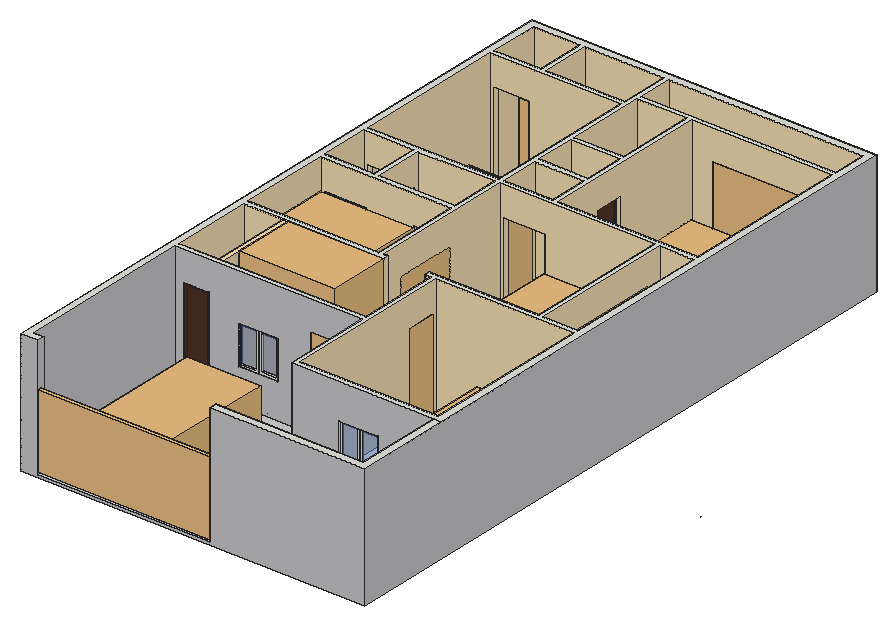
# SketchUp Ruby script. Lengths in inches.
U = 1.inch
M = Sketchup.active_model
def pt(a) = Geom::Point3d.new(a.map { |v| v * U })
def face(e, loops, mat)
  f = e.add_face(loops[0].map { |a| pt(a) })
  loops[1..].each { |l| e.add_face(l.map { |a| pt(a) }).erase! }
  f.material = f.back_material = mat if mat
  f
end
# faces: each face lists its corners as indices into pts; further lists are holes
def faces(e, pts, list, mat = nil) = list.each { |f| face(e, (f[0].is_a?(Array) ? f : [f]).map { |l| l.map { |i| pts[i] } }, mat) }
# xy, xz, yz: faces in a plane at the given z, y or x. An outline is a flat list of corners, or four numbers for a rectangle; further outlines are holes
def ring(l) = l.size == 4 ? [[l[0], l[1]], [l[2], l[1]], [l[2], l[3]], [l[0], l[3]]] : l.each_slice(2).to_a
def flat(e, list, mat, &to3) = list.each { |f| face(e, (f[0].is_a?(Array) ? f : [f]).map { |l| ring(l).map { |u, v| to3.(u, v) } }, mat) }
def xy(e, z, list, mat = nil) = flat(e, list, mat) { |x, y| [x, y, z] }
def xz(e, y, list, mat = nil) = flat(e, list, mat) { |x, z| [x, y, z] }
def yz(e, x, list, mat = nil) = flat(e, list, mat) { |y, z| [x, y, z] }
def lines(e, pts, list) = list.each { |a, b| e.add_line(pt(pts[a]), pt(pts[b])) }
# prism: a flat outline (further loops are holes) pulled along v
def prism(e, loops, v, mat = nil)
  f = face(e, loops, mat); d = Geom::Vector3d.new(v.map { |x| x * U })
  f.pushpull(f.normal.samedirection?(d) ? d.length : -d.length)
end
def box(e, o, s, mat = nil) = prism(e, [[o, [o[0] + s[0], o[1], o[2]], [o[0] + s[0], o[1] + s[1], o[2]], [o[0], o[1] + s[1], o[2]]]], [0, 0, s[2]], mat)
def at(x, y, z, deg = 0) = Geom::Transformation.translation(pt([x, y, z])) * Geom::Transformation.rotation(ORIGIN, Z_AXIS, deg.degrees)
def axes(o, x, y, z) = Geom::Transformation.new([*x, 0, *y, 0, *z, 0, *pt(o).to_a, 1])
def part(name) = M.definitions.add(name)
# library, detail: a bought-in or finely detailed component or shape, given as its bounding box
def library(name, o, s) = part(name).tap { |d| box(d.entities, o, s) }
def detail(e, o, s) = box(e.add_group.entities, o, s)
def put(e, d, t, mat = nil) = e.add_instance(d, t).tap { |i| i.material = mat if mat }
def group(e, t, mat = nil) = e.add_group.tap { |g| g.transformation = t; g.material = mat if mat }.entities
root = M.entities
M.materials.add("Material~26").color = [38, 26, 21]
M.materials.add("Material~5").color = [95, 99, 100]
M.materials.add("Material~69").color = [153, 142, 126]
M.materials.add("Polis06_194").color = [79, 50, 36]
M.materials.add("[0034_Wheat]").color = [245, 222, 179]
M.materials.add("[Carrera Marble]").color = [207, 207, 207]
M.materials.add("[Grass Dark Green]").color = [106, 157, 55]
M.materials.add("[Polished Concrete New]").color = [200, 200, 203]
M.materials.add("[Translucent Glass Blue]").color = [100, 149, 237]
M.materials["[Translucent Glass Blue]"].alpha = 0.5
M.materials.add("[White Square Tile]").color = [240, 234, 230]
M.materials.add("[White Square Tile]1").color = [240, 234, 230]
c1 = library("Return stair",[0,0,0],[148.29,95.17,159.125])
c2 = library("devendra+jangid+[door]+drawings",[57.04,80.03,0],[48,84,6.66])
c3 = library("PINTU+6+YA",[0,-0.6875,0],[35.83,8.07,80.71])
c4 = library("04+Sofa+y+Mesas (1)",[-94.93,-111.67,3.93],[153.81,110.61,64.28])
c5 = library("Glass+Door",[0,0,0],[72,5.22,111.09])
c6 = part("群组\#3")
xy(c6.entities,0,[[0,0,4.72,1.18],[0,34.25,4.72,35.43]],"Polis06_194")
xy(c6.entities,85.26,[[0,1.18,4.72,34.25]],"Polis06_194")
xy(c6.entities,86.61,[[0,0,4.72,35.43]],"Polis06_194")
xz(c6.entities,0,[[0,0,4.72,86.61]],"Polis06_194")
xz(c6.entities,1.18,[[0,0,2.36,85.26],[2.36,0,4.72,85.26]],"Polis06_194")
xz(c6.entities,34.25,[[0,0,4.72,85.26]],"Polis06_194")
xz(c6.entities,35.43,[[0,0,4.72,86.61]],"Polis06_194")
yz(c6.entities,0,[[0,0,1.18,86.61],[34.25,0,35.43,86.61],[1.18,85.26,34.25,86.61]],"Polis06_194")
yz(c6.entities,2.36,[[1.18,0,34.25,0,34.25,85.21,1.18,85.26]],"Polis06_194")
yz(c6.entities,4.72,[[0,0,1.18,86.61],[34.25,0,35.43,86.61],[1.18,85.26,34.25,86.61]],"Polis06_194")
c7 = part("Janela aluminio")
xy(c7.entities,0,[[0,0,47.24,1.57],[23.62,1.57,47.24,2.76],[0,2.76,25.98,3.9375],[0,3.9375,47.24,5.91]])
xy(c7.entities,43.31,[[0,0,47.24,1.57],[23.62,1.57,47.24,2.76],[0,2.76,0,5.91,47.24,5.91,47.24,3.9375,25.98,3.9375,25.98,2.76],[25.98,2.76,47.24,3.9375]])
xz(c7.entities,1.57,[[0,0,23.62,0,23.62,41.34,21.26,41.34,21.26,1.97,1.97,1.97,1.97,41.34,23.62,41.34,23.62,43.31,0,43.31],[[23.62,0,47.24,43.31],[25.7,1.97,45.28,41.34]]])
xz(c7.entities,2.76,[[[0,0,23.62,43.31],[2.36,2.36,21.26,40.94]],[23.62,0,25.98,43.31]])
xz(c7.entities,2.76,[[2.36,2.36,21.26,40.94]],"[Translucent Glass Blue]")
xz(c7.entities,3.9375,[[25.98,0,25.98,2.36,44.88,2.36,44.88,40.94,25.98,40.94,25.98,43.31,47.24,43.31,47.24,0]])
xz(c7.entities,3.9375,[[25.98,2.36,44.88,40.94]],"[Translucent Glass Blue]")
yz(c7.entities,0,[[0,0,1.57,43.31],[2.76,0,5.91,43.31]])
yz(c7.entities,23.62,[[1.57,0,2.76,43.31]])
yz(c7.entities,25.98,[[2.76,0,3.9375,43.31]])
yz(c7.entities,47.24,[[0,0,1.57,43.31],[1.57,0,2.76,43.31],[3.9375,0,5.91,43.31]])
c8 = library("Double bed",[0,0,0],[83.59,95.6,35.43])
c9 = library("2016+Honda+Civic+LX+Sedan",[0.01,0.03,0.02],[16.17,34.46,10.62])
c10 = library("Untitled (9)",[-1.5,0,0],[33.72,42,82.88])
c11 = library("Flower+pot",[-3.29,-4.11,0],[8.25,8.08,16.09])
c12 = library("Group\#38",[0,83.59,1],[18.8125,96.19,84])
c13 = part("3DGeom~69_Defintion\#1")
xy(c13.entities,14.55,[[-498.55,-461.83,498.98,-461.4,-498.98,461.4],[498.98,-461.4,498.55,461.83,-498.98,461.4]],"Material~69")
p = [[-498.55,-461.83,14.55],[-500,-461.99,12.51],[499.14,-462.85,12.51],[498.98,-462.58,13.6875],[498.98,-461.4,14.55],[500,461.99,12.51],
  [-498.98,461.4,14.55],[-499.14,462.85,12.51],[-499.73,-461.83,13.6875],[499.73,461.83,13.6875],[-498.98,462.58,13.6875],[498.55,461.83,14.55]]
faces(c13.entities,p,[[0,1,2],[2,3,0],[4,2,5],[2,4,3],[6,7,1],[1,8,6],[1,0,8],[5,9,4],
  [7,6,10],[11,5,7],[7,10,11],[5,11,9],[3,4,0],[8,0,6],[9,11,4],[10,6,11]],"Material~69")
c14 = part("Group209\#1")
put(c14.entities,c13,axes([-3.37,-15.69,-1.69],[0,-0.13066,0],[0.16609,0,0],[0,0,0.13066]),"Material~69")
c15 = part("Group208\#1")
put(c15.entities,c14,at(0,0,0))
c16 = library("Group74\#1",[-57.27,43.43,23.77],[9.81,9.83,13.8])
c17 = library("Group81\#1",[-36.24,-55.3,0.14],[100.09,119.6,30.24])
c18 = library("Group122\#1",[-22.86,-40.23,0.14],[33.38,47.24,14.48])
c19 = part("3DGeom~26_Defintion\#1")
xz(c19.entities,-351.43,[[-498.73,1.27,498.73,1.27,498.73,43.73],[-498.73,1.27,498.73,43.73,-498.73,43.73]],"Material~26")
xz(c19.entities,291.67,[[-498.73,1.27,-498.73,43.73,498.73,1.27],[498.73,1.27,-498.73,43.73,498.73,43.73]],"Material~26")
yz(c19.entities,-500,[[-350.16,1.27,-350.16,43.73,290.4,1.27],[290.4,1.27,-350.16,43.73,290.4,43.73]],"Material~26")
yz(c19.entities,500,[[-350.16,1.27,290.4,1.27,290.4,43.73],[-350.16,1.27,290.4,43.73,-350.16,43.73]],"Material~26")
p = [[-498.73,-350.16,0],[-498.73,-351.43,1.27],[-500,-350.16,1.27],[-498.73,-350.16,0],[498.73,290.4,0],[498.73,-351.43,1.27],
  [498.73,-351.43,1.27],[-498.73,-351.43,1.27],[-498.73,-350.16,0],[500,-350.16,1.27],[-500,290.4,1.27],[-498.73,291.67,1.27],
  [-498.73,-350.16,0],[-500,-350.16,1.27],[-500,290.4,1.27],[-498.73,-350.16,0],[498.73,290.4,0],[-498.73,-350.16,0],
  [-498.73,291.67,1.27],[500,290.4,1.27],[500,-350.16,1.27],[498.73,290.4,0],[-498.73,291.67,1.27],[498.73,291.67,1.27],
  [498.73,290.4,0],[498.73,291.67,1.27],[500,290.4,1.27],[498.73,290.4,0],[-498.73,-351.43,1.27],[-498.73,-351.43,43.73],
  [-500,-350.16,43.73],[-500,-350.16,43.73],[-500,-350.16,1.27],[-498.73,-351.43,1.27],[500,-350.16,1.27],[500,-350.16,43.73],
  [498.73,-351.43,43.73],[498.73,-351.43,1.27],[-500,290.4,1.27],[-500,290.4,43.73],[-498.73,291.67,43.73],[-498.73,291.67,1.27],
  [498.73,291.67,1.27],[498.73,291.67,43.73],[500,290.4,43.73],[500,290.4,1.27],[498.73,-350.16,45],[-500,-350.16,43.73],
  [-498.73,-351.43,43.73],[-498.73,-351.43,43.73],[498.73,-351.43,43.73],[498.73,-350.16,45],[498.73,-351.43,43.73],[500,-350.16,43.73],
  [498.73,-350.16,45],[-498.73,291.67,43.73],[-500,290.4,43.73],[498.73,-350.16,45],[-500,290.4,43.73],[-500,-350.16,43.73],
  [498.73,-350.16,45],[498.73,291.67,43.73],[-498.73,291.67,43.73],[498.73,-350.16,45],[500,290.4,43.73],[498.73,291.67,43.73],
  [498.73,-350.16,45],[500,-350.16,43.73],[500,290.4,43.73],[498.73,-350.16,45]]
faces(c19.entities,p,[[0,1,2],[3,4,5],[6,7,8],[9,5,4],[10,11,12],[13,14,15],[16,17,18],[19,20,21],
  [22,23,24],[25,26,27],[28,29,30],[31,32,33],[34,35,36],[36,37,34],[38,39,40],[40,41,38],
  [42,43,44],[44,45,42],[46,47,48],[49,50,51],[52,53,54],[55,56,57],[58,59,60],[61,62,63],
  [64,65,66],[67,68,69]],"Material~26")
c20 = part("Group125\#1")
put(c20.entities,c19,axes([-4.62,-16.61,14.625],[0,-0.04724,0],[0.0519,0,0],[0,0,0.04724]),"Material~26")
c21 = part("Group124\#1")
put(c21.entities,c20,at(0,0,0))
c22 = library("Group129\#1",[-11.1,-20.62,16.76],[15.29,19.61,0.96])
c23 = library("Group131\#1",[-0.38,-19.49,16.6875],[3.57,3.64,4.03])
c24 = library("Group133\#1",[-7.61,-17.51,16.58],[9.42,6.3,3.73])
c25 = library("Group141\#1",[-2.9,-28.6875,16.72],[3.31,3.2,9.28])
c26 = library("Group150\#1",[-6.91,-27.56,16.72],[3.31,3.2,9.28])
c27 = library("Group159\#1",[-5.52,-24.1,16.72],[3.31,3.2,7.64])
c28 = library("Group168\#1",[36.22,-65.56,23.76],[3.31,3.19,7.65])
c29 = library("Group177\#1",[29.26,-78.71,0.14],[26.25,21.84,23.61])
c30 = library("Group180\#1",[36.22,-61.78,23.76],[3.31,3.2,7.65])
c31 = library("Group199\#1",[-54.6,36.54,23.82],[10.19,10.22,3.72])
c32 = library("Group204\#1",[42.92,-69.85,23.77],[9.81,9.82,13.8])
c33 = library("Group\#2",[0,-2.58,0],[133.11,142.48,49.27])
c34 = library("Group138\#2",[-7.05,-9.53,17.16],[10,7.13,0.56])
c35 = library("Group135\#2",[-3.38,-9.38,17.65],[5.78,6.62,0.62])
c36 = library("Group\#81",[0,0,0],[96.93,107.95,106.3])
c37 = library("Group\#124",[0,0,0],[71.22,27.85,82.1875])
c38 = library("Group\#145",[0,0,0],[120.6,5.32,84])
xy(root,0,[[0,0,420,780]])
xy(root,3,[[21,0,231,0,231,36.96,219.5625,36.96,219.5625,83.33,231,83.33,231,117,237,117,237,225,234,225,234,202.92,174,202.92,174,225,9,225,9,9,21,9]],"[Carrera Marble]")
xy(root,4,[[219.5625,36.96,231,83.33],[174,202.92,234,208.92]],"[Carrera Marble]")
xy(root,6,[[57,237,63,267],[177.69,330,179.29,330,179.29,332.97],[229.0625,513,276.23,513,279.46,519,240,519,240,525,234,525,234,519,229.0625,519],[381.88,723,389.31,723,392.54,729,381.88,729]])
xy(root,6,[[174,208.92,234,225]],"[Carrera Marble]")
xy(root,6,[[231,9,411,117]],"[Grass Dark Green]")
xy(root,6,[[279.41,117,350.45,123],[[243,123,411,123,411,330,243,330,243,324,237,324,237,330,229.0625,330,229.0625,336,363,336,363,353.23,369,353.23,369,336,411,336,411,513,369,513,369,495.24,363,495.24,363,513,229.0625,513,229.0625,519,234,519,234,525,240,525,240,519,411,519,411,723,381.88,723,381.88,729,411,729,411,771,174,771,174,729,266.46,729,266.46,723,240,723,240,615.73,234,615.73,234,621,228,621,228,627,234,627,234,723,174,723,174,627,198,627,198,621,174,621,174,573,234,573,234,578.84,240,578.84,240,561,234,561,234,567,174,567,174,561,168,561,168,705,55.67,705,55.67,711,66,711,66,717,72,717,72,711,168,711,168,771,72,771,72,747,66,747,66,771,9,771,9,711,13.3,711,13.3,705,9,705,9,519,13.31,519,13.31,513,9,513,9,453,13.2,453,13.2,447,9,447,9,336,168,336,168,362.92,174,362.92,174,336,179.29,336,179.29,330,63,330,63,231,174,231,174,225,234,225,234,231,237,231,237,288,243,288],[168,436.64,168,447,160.04,447,160.04,453,168,453,168,513,75,513,75,506.98,69,506.98,69,513,64.32,513,64.32,519,168,519,168,525,174,525,174,519,179.29,519,179.29,513,174,513,174,436.64],[64.32,447,64.32,453,69,453,69,457.49,75,457.49,75,453,122.37,453,122.37,447]],[57,231,63,237],[57,267,63,330]],"[White Square Tile]")
xy(root,6,[[19.95,225,49.95,225,49.95,231,57,231,57,330,9,330,9,231,19.95,231]],"[White Square Tile]1")
xy(root,45.1875,[[85.93,225,133.93,231]],"[Polished Concrete New]")
xy(root,58.77,[[294.94,117,342.94,123]],"[Polished Concrete New]")
xy(root,75.83,[[0,470.52,9,494.52]],"[Polished Concrete New]")
xy(root,93.1875,[[85.93,225,133.93,231]],"[Polished Concrete New]")
xy(root,99.83,[[0,470.52,9,494.52]],"[Polished Concrete New]")
xy(root,106.77,[[294.94,117,342.94,123]],"[Polished Concrete New]")
xy(root,114,[[19.95,225,49.95,231],[174,225,234,231],[57,237,63,267],[237,288,243,324],[363,353.23,369,495.24],
  [168,362.92,174,436.64],[13.2,447,64.32,453],[122.37,447,160.04,453],[179.29,513,229.0625,519],[168,525,174,561],
  [234,525,240,561],[234,578.84,240,615.73],[198,621,228,627],[13.3,705,55.67,711],[66,717,72,747],
  [266.46,723,381.88,729]])
xy(root,114,[[69,457.49,75,506.98],[13.31,513,64.32,519]],"[0034_Wheat]")
xy(root,150,[[[0,0,21,0,21,9,9,9,9,225,237,225,237,117,420,117,420,780,0,780],[9,231,9,330,179.29,330,179.29,336,174,336,174,513,363,513,363,336,229.0625,336,229.0625,330,237,330,237,231],[240,519,411,723],[243,123,411,330],[9,519,168,705],[9,336,168,447],[174,729,411,771],[369,336,411,513],[174,627,234,723],[72,711,168,771],[75,453,168,513],[9,453,69,513],[9,711,66,771],[174,519,234,567],[174,573,234,621]],[231,0,420,0,420,117,411,117,411,9,231,9]])
xy(root,150,[[57,231,63,330]],"[0034_Wheat]")
xz(root,0,[[0,0,420,0,420,150,231,150,231,3,21,3,21,150,0,150]],"[Polished Concrete New]")
xz(root,9,[[9,3,21,150],[231,6,411,150]],"[Polished Concrete New]")
xz(root,36.96,[[219.5625,3,231,4]],"[Carrera Marble]")
xz(root,83.33,[[219.5625,3,231,4]],"[Carrera Marble]")
xz(root,117,[[231,3,237,6]],"[Carrera Marble]")
xz(root,117,[[[237,6,411,150],[294.94,58.77,342.94,106.77]]],"[Polished Concrete New]")
xz(root,123,[[[243,6,411,150],[294.94,58.77,342.94,106.77]]],"[0034_Wheat]")
xz(root,202.92,[[174,3,234,4]],"[Carrera Marble]")
xz(root,208.92,[[174,4,234,6]],"[Carrera Marble]")
xz(root,225,[[[9,3,174,3,174,114,234,114,234,3,237,3,237,150,9,150],[19.95,6,49.95,114],[85.93,45.1875,133.93,93.1875]]],"[Polished Concrete New]")
xz(root,231,[[9,6,9,150,57,150,57,6,49.95,6,49.95,114,19.95,114,19.95,6],[57,6,63,150],[[63,6,63,150,237,150,237,6,234,6,234,114,174,114,174,6],[85.93,45.1875,133.93,93.1875]]],"[0034_Wheat]")
xz(root,237,[[57,6,63,114]],"[0034_Wheat]")
xz(root,267,[[57,6,63,114]],"[0034_Wheat]")
xz(root,288,[[237,6,243,114]],"[0034_Wheat]")
xz(root,324,[[237,6,243,114]],"[0034_Wheat]")
xz(root,330,[[9,6,57,150],[57,6,63,150],[63,6,179.29,150],[229.0625,6,237,150],[243,6,411,150]],"[0034_Wheat]")
xz(root,336,[[9,6,168,150],[174,6,179.29,150],[229.0625,6,363,150],[369,6,411,150]],"[0034_Wheat]")
xz(root,353.23,[[363,6,369,114]],"[0034_Wheat]")
xz(root,362.92,[[168,6,174,114]],"[0034_Wheat]")
xz(root,436.64,[[168,6,174,114]],"[0034_Wheat]")
xz(root,447,[[9,6,13.2,6,13.2,114,64.32,114,64.32,6,122.37,6,122.37,114,160.04,114,160.04,6,168,6,168,150,9,150]],"[0034_Wheat]")
xz(root,453,[[9,6,9,150,69,150,69,6,64.32,6,64.32,114,13.2,114,13.2,6],[75,6,75,150,168,150,168,6,160.04,6,160.04,114,122.37,114,122.37,6]],"[0034_Wheat]")
xz(root,457.49,[[69,6,75,114]],"[0034_Wheat]")
xz(root,470.52,[[0,75.83,9,99.83]],"[Polished Concrete New]")
xz(root,494.52,[[0,75.83,9,99.83]],"[Polished Concrete New]")
xz(root,495.24,[[363,6,369,114]],"[0034_Wheat]")
xz(root,506.98,[[69,6,75,114]],"[0034_Wheat]")
xz(root,513,[[9,6,13.31,6,13.31,114,64.32,114,64.32,6,69,6,69,150,9,150],[75,6,168,150],[174,6,179.29,6,179.29,114,229.0625,114,229.0625,6,363,6,363,150,174,150],[369,6,411,150]],"[0034_Wheat]")
xz(root,519,[[9,6,9,150,168,150,168,6,64.32,6,64.32,114,13.31,114,13.31,6],[174,6,174,150,234,150,234,6,229.0625,6,229.0625,114,179.29,114,179.29,6],[240,6,411,150]],"[0034_Wheat]")
xz(root,525,[[168,6,174,114],[234,6,240,114]],"[0034_Wheat]")
xz(root,561,[[168,6,174,114],[234,6,240,114]],"[0034_Wheat]")
xz(root,567,[[174,6,234,150]],"[0034_Wheat]")
xz(root,573,[[174,6,234,150]],"[0034_Wheat]")
xz(root,578.84,[[234,6,240,114]],"[0034_Wheat]")
xz(root,615.73,[[234,6,240,114]],"[0034_Wheat]")
xz(root,621,[[174,6,198,6,198,114,228,114,228,6,234,6,234,150,174,150]],"[0034_Wheat]")
xz(root,627,[[174,6,174,150,234,150,234,6,228,6,228,114,198,114,198,6]],"[0034_Wheat]")
xz(root,705,[[9,6,13.3,6,13.3,114,55.67,114,55.67,6,168,6,168,150,9,150]],"[0034_Wheat]")
xz(root,711,[[9,6,9,150,66,150,66,6,55.67,6,55.67,114,13.3,114,13.3,6],[72,6,168,150]],"[0034_Wheat]")
xz(root,717,[[66,6,72,114]],"[0034_Wheat]")
xz(root,723,[[174,6,234,150],[240,6,266.46,6,266.46,114,381.88,114,381.88,6,411,6,411,150,240,150]],"[0034_Wheat]")
xz(root,729,[[174,6,174,150,411,150,411,6,381.88,6,381.88,114,266.46,114,266.46,6]],"[0034_Wheat]")
xz(root,747,[[66,6,72,114]],"[0034_Wheat]")
xz(root,771,[[9,6,66,150],[72,6,168,150],[174,6,411,150]],"[0034_Wheat]")
xz(root,780,[[0,0,420,150]],"[Polished Concrete New]")
yz(root,0,[[[0,0,780,150],[470.52,75.83,494.52,99.83]]],"[Polished Concrete New]")
yz(root,9,[[231,6,330,150],[336,6,447,150],[[453,6,513,150],[470.52,75.83,494.52,99.83]],[519,6,705,150],[711,6,771,150]],"[0034_Wheat]")
yz(root,9,[[9,3,225,150]],"[Polished Concrete New]")
yz(root,13.2,[[447,6,453,114]],"[0034_Wheat]")
yz(root,13.3,[[705,6,711,114]],"[0034_Wheat]")
yz(root,13.31,[[513,6,519,114]],"[0034_Wheat]")
yz(root,19.95,[[225,6,231,114]],"[0034_Wheat]")
yz(root,21,[[0,3,9,150]],"[Polished Concrete New]")
yz(root,49.95,[[225,6,231,114]],"[0034_Wheat]")
yz(root,55.67,[[705,6,711,114]],"[0034_Wheat]")
yz(root,57,[[231,6,231,150,330,150,330,6,267,6,267,114,237,114,237,6]],"[0034_Wheat]")
yz(root,63,[[231,6,231,150,330,150,330,6,267,6,267,114,237,114,237,6]],"[0034_Wheat]")
yz(root,64.32,[[447,6,453,114],[513,6,519,114]],"[0034_Wheat]")
yz(root,66,[[711,6,711,150,771,150,771,6,747,6,747,114,717,114,717,6]],"[0034_Wheat]")
yz(root,69,[[453,6,453,150,513,150,513,6,506.98,6,506.98,114,457.49,114,457.49,6]],"[0034_Wheat]")
yz(root,72,[[711,6,717,6,717,114,747,114,747,6,771,6,771,150,711,150]],"[0034_Wheat]")
yz(root,75,[[453,6,457.49,6,457.49,114,506.98,114,506.98,6,513,6,513,150,453,150]],"[0034_Wheat]")
yz(root,85.93,[[225,45.1875,231,93.1875]],"[Polished Concrete New]")
yz(root,122.37,[[447,6,453,114]],"[0034_Wheat]")
yz(root,133.93,[[225,45.1875,231,93.1875]],"[Polished Concrete New]")
yz(root,160.04,[[447,6,453,114]],"[0034_Wheat]")
yz(root,168,[[336,6,336,150,447,150,447,6,436.64,6,436.64,114,362.92,114,362.92,6],[453,6,513,150],[519,6,519,150,705,150,705,6,561,6,561,114,525,114,525,6],[711,6,771,150]],"[0034_Wheat]")
yz(root,174,[[225,6,231,114],[336,6,362.92,6,362.92,114,436.64,114,436.64,6,513,6,513,150,336,150],[519,6,525,6,525,114,561,114,561,6,567,6,567,150,519,150],[573,6,621,150],[627,6,723,150],
  [729,6,771,150]],"[0034_Wheat]")
yz(root,174,[[202.92,3,208.92,4],[208.92,3,225,6]],"[Carrera Marble]")
yz(root,179.29,[[330,6,336,150],[513,6,519,114]],"[0034_Wheat]")
yz(root,198,[[621,6,627,114]],"[0034_Wheat]")
yz(root,219.5625,[[36.96,3,83.33,4]],"[Carrera Marble]")
yz(root,228,[[621,6,627,114]],"[0034_Wheat]")
yz(root,229.0625,[[330,6,336,150],[513,6,519,114]],"[0034_Wheat]")
yz(root,231,[[0,3,0,150,9,150,9,6,117,6,117,3,83.33,3,83.33,4,36.96,4,36.96,3]],"[Polished Concrete New]")
yz(root,234,[[225,6,231,114],[519,6,519,150,567,150,567,6,561,6,561,114,525,114,525,6],[573,6,573,150,621,150,621,6,615.73,6,615.73,114,578.84,114,578.84,6],[627,6,723,150]],"[0034_Wheat]")
yz(root,234,[[202.92,3,208.92,4],[208.92,3,225,6]],"[Carrera Marble]")
yz(root,237,[[231,6,231,150,330,150,330,6,324,6,324,114,288,114,288,6]],"[0034_Wheat]")
yz(root,237,[[117,3,225,150]],"[Polished Concrete New]")
yz(root,240,[[519,6,525,6,525,114,561,114,561,6,578.84,6,578.84,114,615.73,114,615.73,6,723,6,723,150,519,150]],"[0034_Wheat]")
yz(root,243,[[123,6,288,6,288,114,324,114,324,6,330,6,330,150,123,150]],"[0034_Wheat]")
yz(root,266.46,[[723,6,729,114]],"[0034_Wheat]")
yz(root,294.94,[[117,58.77,123,106.77]],"[Polished Concrete New]")
yz(root,342.94,[[117,58.77,123,106.77]],"[Polished Concrete New]")
yz(root,363,[[336,6,336,150,513,150,513,6,495.24,6,495.24,114,353.23,114,353.23,6]],"[0034_Wheat]")
yz(root,369,[[336,6,353.23,6,353.23,114,495.24,114,495.24,6,513,6,513,150,336,150]],"[0034_Wheat]")
yz(root,381.88,[[723,6,729,114]],"[0034_Wheat]")
yz(root,411,[[123,6,330,150],[336,6,513,150],[519,6,723,150],[729,6,771,150]],"[0034_Wheat]")
yz(root,411,[[9,6,117,150]],"[Polished Concrete New]")
yz(root,420,[[0,0,780,150]],"[Polished Concrete New]")
p = [[266.18,117,6],[266.18,123,6],[243,171,114],[237,171,114],[568.47,325.94,6],[568.47,326.94,6],
  [567.47,326.94,6],[121.15,225,6],[124.38,231,6],[411,763.29,6],[420,780,6],[-382.04,-117.92,0],
  [-382.04,-117.92,4.0625]]
lines(root,p,[[0,1],[2,3],[4,5],[5,6],[6,4],[7,8],[9,10],[11,12]])
put(root,c1,axes([63,254.8125,6],[0.7842,0,0],[0,0.79,0],[0,0,0.90495]))
put(root,c2,axes([102.7,231.66,-96.9],[1.25,0,0],[0,0,1.28571],[0,-1,0]))
put(root,c3,axes([168,561,6],[0,-1.00475,0],[1,0,0],[0,0,1.33815]))
put(root,c4,axes([308.85,513.86,2.07],[0.85118,0,0],[0,0.8165,0],[0,0,1]))
put(root,c5,axes([266.46,723,6],[1.60308,0,0],[0,1,0],[0,0,0.97215]))
put(root,c6,axes([49.95,225,6],[0,1,0],[-0.84667,0,0],[0,0,1.24691]))
put(root,c7,axes([294.94,117,58.77],[1.016,0,0],[0,1,0],[0,0,1.10836]))
put(root,c8,at(92.59,673.23,6,180))
put(root,c8,at(323.59,722.6,6,180))
put(root,c6,axes([70.72,747,6],[-1,0,0],[0,-0.84667,0],[0,0,1.24691]))
put(root,c6,axes([198,625.72,6],[0,-1,0],[0.84667,0,0],[0,0,1.24691]))
put(root,c3,axes([234,561,6],[0,-1.00475,0],[1,0,0],[0,0,1.33815]))
put(root,c3,axes([237,324,6],[0,-1.00475,0],[1,0,0],[0,0,1.33815]))
put(root,c5,axes([363,495.24,6],[0,-1.97232,0],[1,0,0],[0,0,0.97215]))
put(root,c5,axes([174,362.92,6],[0,1.02389,0],[-1,0,0],[0,0,0.97215]))
put(root,c6,axes([63,267,6],[-1,0,0],[0,-0.84667,0],[0,0,1.24691]))
put(root,c7,axes([85.93,225,45.1875],[1.016,0,0],[0,1,0],[0,0,1.10836]))
put(root,c7,axes([0,494.52,75.83],[0,-0.508,0],[1,0,0],[0,0,0.55418]))
put(root,c9,axes([141.51,189.41,5.89],[-5.55235,0,0],[0,-4.88592,0],[0,0,5.06788]))
put(root,c10,at(16.91,771.24,6,-90))
put(root,c10,at(173.76,575.65,6))
put(root,c11,axes([391.89,494.66,6],[2.108,0,0],[0,2.6691,0],[0,0,2]))
put(root,c11,axes([391.89,354.53,6],[2.108,0,0],[0,2.6691,0],[0,0,2]))
put(root,c11,axes([385.04,751.53,6],[2.108,0,0],[0,2.6691,0],[0,0,2]))
put(root,c11,axes([189.54,751.53,6],[2.108,0,0],[0,2.6691,0],[0,0,2]))
put(root,c11,axes([391.89,96.84,6],[2.108,0,0],[0,2.6691,0],[0,0,2]))
put(root,c11,axes([391.89,62.59,6],[2.108,0,0],[0,2.6691,0],[0,0,2]))
put(root,c11,axes([391.89,29.84,6],[2.108,0,0],[0,2.6691,0],[0,0,2]))
put(root,c11,axes([357.01,29.84,6],[2.108,0,0],[0,2.6691,0],[0,0,2]))
put(root,c11,axes([322.26,29.84,6],[2.108,0,0],[0,2.6691,0],[0,0,2]))
put(root,c11,axes([287.32,29.84,6],[2.108,0,0],[0,2.6691,0],[0,0,2]))
put(root,c11,axes([254.39,29.84,6],[2.108,0,0],[0,2.6691,0],[0,0,2]))
put(root,c12,at(424.08,336,5,90))
put(root,c15,axes([349.18,273.56,6.06],[0.84099,0,0],[0,0.8778,0],[0,0,1]))
put(root,c16,axes([349.18,273.56,6.06],[0.84099,0,0],[0,0.8778,0],[0,0,1]))
put(root,c17,axes([349.18,273.56,6.06],[0.84099,0,0],[0,0.8778,0],[0,0,1]),"Material~5")
put(root,c18,axes([349.18,273.56,6.06],[0.84099,0,0],[0,0.8778,0],[0,0,1]))
put(root,c21,axes([349.18,273.56,6.06],[0.84099,0,0],[0,0.8778,0],[0,0,1]))
put(root,c22,axes([349.18,273.56,6.06],[0.84099,0,0],[0,0.8778,0],[0,0,1]))
put(root,c23,axes([349.18,273.56,6.06],[0.84099,0,0],[0,0.8778,0],[0,0,1]))
put(root,c24,axes([349.18,273.56,6.06],[0.84099,0,0],[0,0.8778,0],[0,0,1]))
put(root,c25,axes([349.18,273.56,6.06],[0.84099,0,0],[0,0.8778,0],[0,0,1]))
put(root,c26,axes([349.18,273.56,6.06],[0.84099,0,0],[0,0.8778,0],[0,0,1]))
put(root,c27,axes([349.18,273.56,6.06],[0.84099,0,0],[0,0.8778,0],[0,0,1]))
put(root,c28,axes([349.18,273.56,6.06],[0.84099,0,0],[0,0.8778,0],[0,0,1]))
put(root,c29,axes([349.18,273.56,6.06],[0.84099,0,0],[0,0.8778,0],[0,0,1]))
put(root,c30,axes([349.18,273.56,6.06],[0.84099,0,0],[0,0.8778,0],[0,0,1]))
put(root,c31,axes([349.18,273.56,6.06],[0.84099,0,0],[0,0.8778,0],[0,0,1]))
put(root,c32,axes([349.18,273.56,6.06],[0.84099,0,0],[0,0.8778,0],[0,0,1]))
put(root,c33,axes([296.23,210.76,6.19],[0.79096,0,0],[0,0.82557,0],[0,0,0.9405]))
put(root,c34,axes([348.77,273.26,5.01],[0.89357,0,0],[0,0.93268,0],[0,0,1.06252]),"Material~5")
put(root,c35,axes([348.77,273.26,5.01],[0.89357,0,0],[0,0.93268,0],[0,0,1.06252]),"Material~5")
put(root,c36,axes([9,336,6],[1.17,0,0],[0,1.02826,0],[0,0,1]))
put(root,c37,at(234,643.62,6,90))
put(root,c37,at(83.875,711,6))
put(root,c37,at(9,316.68,6,-90))
put(root,c38,axes([231,5.32,6],[-1.74129,0,0],[0,-1,0],[0,0,1.07]))
